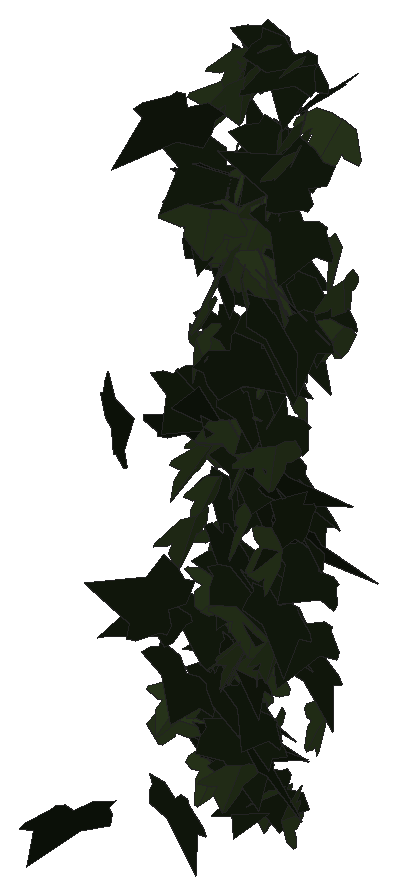
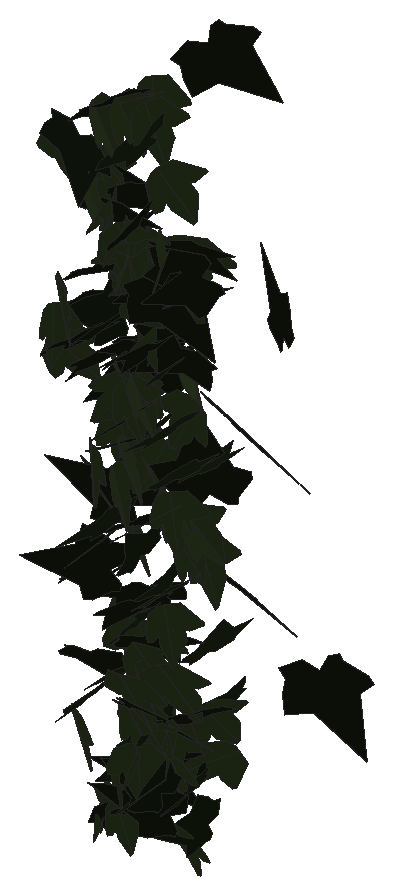
# SketchUp Ruby script. Lengths in inches.
U = 1.inch
M = Sketchup.active_model
def pt(a) = Geom::Point3d.new(a.map { |v| v * U })
def face(e, loops, mat)
  f = e.add_face(loops[0].map { |a| pt(a) })
  loops[1..].each { |l| e.add_face(l.map { |a| pt(a) }).erase! }
  f.material = f.back_material = mat if mat
  f
end
# faces: each face lists its corners as indices into pts; further lists are holes
def faces(e, pts, list, mat = nil) = list.each { |f| face(e, (f[0].is_a?(Array) ? f : [f]).map { |l| l.map { |i| pts[i] } }, mat) }
# xy, xz, yz: faces in a plane at the given z, y or x. An outline is a flat list of corners, or four numbers for a rectangle; further outlines are holes
def ring(l) = l.size == 4 ? [[l[0], l[1]], [l[2], l[1]], [l[2], l[3]], [l[0], l[3]]] : l.each_slice(2).to_a
def flat(e, list, mat, &to3) = list.each { |f| face(e, (f[0].is_a?(Array) ? f : [f]).map { |l| ring(l).map { |u, v| to3.(u, v) } }, mat) }
def xy(e, z, list, mat = nil) = flat(e, list, mat) { |x, y| [x, y, z] }
def xz(e, y, list, mat = nil) = flat(e, list, mat) { |x, z| [x, y, z] }
def yz(e, x, list, mat = nil) = flat(e, list, mat) { |y, z| [x, y, z] }
def lines(e, pts, list) = list.each { |a, b| e.add_line(pt(pts[a]), pt(pts[b])) }
# prism: a flat outline (further loops are holes) pulled along v
def prism(e, loops, v, mat = nil)
  f = face(e, loops, mat); d = Geom::Vector3d.new(v.map { |x| x * U })
  f.pushpull(f.normal.samedirection?(d) ? d.length : -d.length)
end
def box(e, o, s, mat = nil) = prism(e, [[o, [o[0] + s[0], o[1], o[2]], [o[0] + s[0], o[1] + s[1], o[2]], [o[0], o[1] + s[1], o[2]]]], [0, 0, s[2]], mat)
def at(x, y, z, deg = 0) = Geom::Transformation.translation(pt([x, y, z])) * Geom::Transformation.rotation(ORIGIN, Z_AXIS, deg.degrees)
def axes(o, x, y, z) = Geom::Transformation.new([*x, 0, *y, 0, *z, 0, *pt(o).to_a, 1])
def part(name) = M.definitions.add(name)
# library, detail: a bought-in or finely detailed component or shape, given as its bounding box
def library(name, o, s) = part(name).tap { |d| box(d.entities, o, s) }
def detail(e, o, s) = box(e.add_group.entities, o, s)
def put(e, d, t, mat = nil) = e.add_instance(d, t).tap { |i| i.material = mat if mat }
def group(e, t, mat = nil) = e.add_group.tap { |g| g.transformation = t; g.material = mat if mat }.entities
root = M.entities
M.materials.add("1026 AP 7946 SUNNY SIDE UP").color = [254, 231, 186]
M.materials.add("efeu1").color = [18, 25, 13]
M.materials.add("efeu2").color = [43, 57, 29]
c1 = part("ivyleaf_9")
p = [[1.54,2.16,1.25],[1.36,2.04,1.19],[-0.21,0.99,0.68],[-0.71,1.11,0.82],[-0.85,0.86,0.67],[-0.8,0.17,0.21],
  [-0.9,-0.01,0.1],[-0.67,-0.16,-0.02],[-0.08,-0.08,-0.05],[-0.03,-0.6,-0.4],[0.65,-0.88,-0.66],[0.83,-0.6,-0.49],
  [1.29,-0.42,-0.43],[1.8125,-0.07,-0.26],[1.21,0.44,0.15]]
faces(c1.entities,p,[[0,1,2,3,4,5,6,7,8,9,10,11,12,13,14]],"efeu1")
c2 = part("ivyleaf_10")
p = [[0,0.5,-0.03],[-0.0625,2.02,-0.43],[-0.19,2.01,-0.46],[-0.54,1.05,-0.29],[-0.52,0.625,-0.18],[-0.83,0.76,-0.28],
  [-1.16,0.64,-0.33],[-1.15,0.33,-0.24],[-0.77,-0.39,0.02],[-0.3,-0.51,0.16],[0.04,-0.48,0.23],[-0.02,2.01,-0.4375],
  [-0.06,2.01,-0.43],[0.04,-0.49,0.23],[0.67,-0.49,0.14],[1.38,0.36,-0.2],[1.375,0.51,-0.24],[0.81,0.65,-0.19],
  [0.62,0.59,-0.15],[0.6,1.09,-0.28],[0.5,1.23,-0.31]]
faces(c2.entities,p,[[0,1,2,3,4,5,6,7,8,9,10],[11,12,0,13,14,15,16,17,18,19,20]],"efeu2")
put(root,c1,axes([112.36,212.67,281.68],[-0.13343,-0.31321,-0.01587],[0.0925,-0.00204,-0.32907],[0.4842,-0.08592,0.05849]),"1026 AP 7946 SUNNY SIDE UP")
put(root,c1,axes([112.74,212.8,288.39],[0.08903,0.21961,-0.26711],[-0.18165,-0.23608,-0.23226],[-0.50404,0.12387,0.03652]),"1026 AP 7946 SUNNY SIDE UP")
put(root,c2,axes([112.77,212.73,282.15],[-0.39871,-0.07954,0.18483],[-0.22985,-0.12011,-0.26772],[0.20687,-0.28675,0.05877]),"1026 AP 7946 SUNNY SIDE UP")
put(root,c1,axes([112.28,212.46,279.84],[0.33832,-0.23015,0.04396],[0.03121,-0.04159,-0.32451],[0.36711,0.21563,-0.01292]),"1026 AP 7946 SUNNY SIDE UP")
put(root,c2,axes([112.625,212.23,284.41],[0.02229,-0.31208,0.16445],[-0.00199,-0.16158,-0.32269],[0.55246,0.01201,-0.0078]),"1026 AP 7946 SUNNY SIDE UP")
put(root,c1,axes([112.59,212.19,285.28],[-0.22713,-0.19626,0.23409],[-0.02446,-0.24806,-0.23123],[0.47281,-0.10711,0.10049]),"1026 AP 7946 SUNNY SIDE UP")
put(root,c1,axes([112.8,212.52,288.93],[-0.49151,-0.14511,0.04267],[-0.03788,-0.04796,-0.35367],[0.2346,-0.31176,0.03228]),"1026 AP 7946 SUNNY SIDE UP")
put(root,c1,axes([112.56,212.62,288.16],[-0.17816,-0.31965,0.08154],[0.00298,-0.08624,-0.34854],[0.51848,-0.10934,0.03002]),"1026 AP 7946 SUNNY SIDE UP")
put(root,c1,axes([112.32,212.57,288.63],[0.5129,0.04063,0.11681],[0.17107,0.03949,-0.33748],[-0.08046,0.34299,0.02707]),"1026 AP 7946 SUNNY SIDE UP")
put(root,c1,axes([112.39,212.91,287.62],[-0.19443,-0.09617,-0.31279],[0.42257,0.14219,-0.15861],[0.26723,-0.29483,0.02323]),"1026 AP 7946 SUNNY SIDE UP")
put(root,c2,axes([112.74,212.74,283.11],[-0.1662,-0.30756,-0.00442],[0.01182,0.00011,-0.33495],[0.48347,-0.10573,0.00667]),"1026 AP 7946 SUNNY SIDE UP")
put(root,c1,axes([112.48,212.63,280.35],[0.11231,-0.30109,0.06167],[0.01182,-0.06148,-0.31907],[0.48308,0.0715,-0.00653]),"1026 AP 7946 SUNNY SIDE UP")
put(root,c1,axes([112.51,212.91,287.31],[0.02358,-0.30949,0.14387],[0.00979,-0.14128,-0.32004],[0.53495,0.01623,-0.00048]),"1026 AP 7946 SUNNY SIDE UP")
put(root,c1,axes([112.59,212,284.89],[0.47331,0.11972,0.15524],[-0.23704,-0.02521,0.33221],[0.18678,-0.33537,0.02822]),"1026 AP 7946 SUNNY SIDE UP")
put(root,c2,axes([112.84,212.63,290.03],[-0.14622,-0.30283,0.16471],[-0.04767,-0.15953,-0.32688],[0.53763,-0.09651,0.01581]),"1026 AP 7946 SUNNY SIDE UP")
put(root,c2,axes([112.52,211.7,280.51],[-0.14499,-0.12302,-0.29264],[0.36185,0.16992,-0.15215],[0.32404,-0.24479,0.03897]),"1026 AP 7946 SUNNY SIDE UP")
put(root,c2,axes([112.87,212.82,288.15],[-0.50464,-0.10978,0.06791],[-0.07296,-0.06786,-0.34627],[0.18821,-0.32066,0.04785]),"1026 AP 7946 SUNNY SIDE UP")
put(root,c2,axes([112.76,212.4,279.51],[0.42028,-0.18104,0.00491],[-0.01497,-0.02436,-0.33168],[0.28442,0.26624,-0.02472]),"1026 AP 7946 SUNNY SIDE UP")
put(root,c2,axes([112.72,212.27,286.22],[-0.44572,0.16772,-0.0709],[0.07739,-0.05357,-0.33896],[-0.27495,-0.28697,0.01953]),"1026 AP 7946 SUNNY SIDE UP")
put(root,c2,axes([112.84,212.49,284.77],[-0.17448,-0.31481,-0.02675],[0.01254,0.02282,-0.34374],[0.49631,-0.11125,-0.00072]),"1026 AP 7946 SUNNY SIDE UP")
put(root,c1,axes([112.53,212.83,286.27],[0.22125,-0.29308,-0.08379],[0.02449,0.09466,-0.32982],[0.47694,0.1311,0.05581]),"1026 AP 7946 SUNNY SIDE UP")
put(root,c1,axes([112.68,212.62,285.32],[-0.15085,-0.26183,0.18911],[0.03789,-0.1985,-0.27763],[0.50272,-0.06361,0.07767]),"1026 AP 7946 SUNNY SIDE UP")
put(root,c2,axes([112.87,211.6,281.01],[-0.16942,-0.22258,0.21145],[0.01315,-0.22123,-0.24243],[0.47725,-0.07292,0.08175]),"1026 AP 7946 SUNNY SIDE UP")
put(root,c2,axes([112.82,212.24,283.99],[0.01482,-0.29803,0.14397],[0.05323,-0.13988,-0.30678],[0.51599,0.02299,0.02751]),"1026 AP 7946 SUNNY SIDE UP")
put(root,c2,axes([112.78,212.74,287.64],[0.12285,0.33519,-0.00481],[-0.04975,0.00065,-0.35313],[-0.52481,0.0784,0.03235]),"1026 AP 7946 SUNNY SIDE UP")
put(root,c2,axes([112.8125,212.39,281.07],[-0.03901,-0.28735,-0.15112],[0.0832,0.13987,-0.29394],[0.49926,-0.04576,0.03718]),"1026 AP 7946 SUNNY SIDE UP")
put(root,c2,axes([112.9,211.7,283.66],[-0.06475,-0.38216,0.00443],[0.00721,-0.007,-0.39598],[0.60096,-0.04109,0.00523]),"1026 AP 7946 SUNNY SIDE UP")
put(root,c1,axes([112.74,212.9,283.53],[-0.10918,-0.28482,0.14106],[0.01352,-0.14348,-0.30027],[0.49785,-0.05857,0.03909]),"1026 AP 7946 SUNNY SIDE UP")
put(root,c2,axes([112.78,212.87,288.83],[-0.01932,0.08766,-0.34444],[0.04851,-0.33344,-0.09304],[-0.54208,-0.03296,0.00395]),"1026 AP 7946 SUNNY SIDE UP")
put(root,c1,axes([113.07,208.88,280.4],[-0.0023,0.33109,-0.24619],[0.00828,-0.24082,-0.34249],[-0.64374,-0.00428,-0.00353]),"1026 AP 7946 SUNNY SIDE UP")
put(root,c2,axes([112.92,212.51,280.7],[0.44827,-0.14908,0.0037],[-0.01323,-0.02564,-0.33044],[0.23415,0.28396,-0.02576]),"1026 AP 7946 SUNNY SIDE UP")
put(root,c1,axes([113.25,210.88,282.83],[-0.51994,0.12954,0.00606],[-0.0273,-0.03027,-0.3643],[-0.20201,-0.32932,0.03363]),"1026 AP 7946 SUNNY SIDE UP")
put(root,c1,axes([112.75,212.99,287.59],[0.04721,-0.31808,-0.11947],[0.02888,0.11597,-0.32724],[0.53059,0.02199,0.02844]),"1026 AP 7946 SUNNY SIDE UP")
put(root,c1,axes([113.31,212.83,281.53],[-0.46194,0.07247,0.09364],[-0.15939,-0.04098,-0.30548],[-0.08845,-0.30465,0.06145]),"1026 AP 7946 SUNNY SIDE UP")
put(root,c2,axes([113.09,211.87,288.5],[-0.44664,-0.19902,0.03307],[-0.0182,-0.04122,-0.35646],[0.31676,-0.283,0.02615]),"1026 AP 7946 SUNNY SIDE UP")
put(root,c2,axes([112.83,212.04,286.34],[-0.08709,-0.11489,-0.34524],[0.15181,-0.3306,0.09859],[-0.53497,-0.07511,0.08418]),"1026 AP 7946 SUNNY SIDE UP")
put(root,c2,axes([113.1875,212.74,281.46],[0.46257,-0.06588,-0.12299],[-0.17817,0.03822,-0.31011],[0.11836,0.31503,0.01386]),"1026 AP 7946 SUNNY SIDE UP")
put(root,c1,axes([112.97,212.94,287.47],[-0.21006,-0.28712,-0.12868],[0.12665,0.09789,-0.32425],[0.47472,-0.15317,0.02957]),"1026 AP 7946 SUNNY SIDE UP")
put(root,c1,axes([113.16,212.69,282.625],[-0.35266,-0.23229,0.00647],[0.01705,-0.02101,-0.33197],[0.36505,-0.22342,0.02175]),"1026 AP 7946 SUNNY SIDE UP")
put(root,c1,axes([112.74,212.75,279.98],[0.26936,-0.0773,0.26366],[0.34164,-0.13775,-0.19316],[0.24608,0.27585,-0.02043]),"1026 AP 7946 SUNNY SIDE UP")
put(root,c1,axes([112.79,212.88,280.375],[0.19172,-0.17623,0.23619],[0.2556,-0.16532,-0.21998],[0.37757,0.2014,0.02899]),"1026 AP 7946 SUNNY SIDE UP")
put(root,c2,axes([113.22,212.82,280.78],[-0.31728,-0.24219,0.01756],[0.01614,-0.03243,-0.3236],[0.38158,-0.20001,0.02828]),"1026 AP 7946 SUNNY SIDE UP")
put(root,c1,axes([112.95,212.12,281.08],[0.15516,-0.30173,-0.06711],[-0.00335,0.06593,-0.32612],[0.4848,0.09702,0.01923]),"1026 AP 7946 SUNNY SIDE UP")
put(root,c2,axes([113.24,212.48,290.85],[-0.12212,-0.35072,0.04215],[-0.00261,-0.04356,-0.37024],[0.55559,-0.0773,0.00753]),"1026 AP 7946 SUNNY SIDE UP")
put(root,c2,axes([113.28,212.65,282.32],[-0.12128,-0.27246,0.15403],[-0.02122,-0.15256,-0.29145],[0.4894,-0.07414,0.02553]),"1026 AP 7946 SUNNY SIDE UP")
put(root,c1,axes([113.04,212.92,280.25],[0.01083,-0.29283,0.11314],[0.01812,-0.1112,-0.30229],[0.49236,0.01053,0.00864]),"1026 AP 7946 SUNNY SIDE UP")
put(root,c2,axes([113.27,212.93,281.94],[0.46364,-0.07499,-0.09593],[-0.14041,0.02492,-0.31328],[0.12422,0.30808,0.00392]),"1026 AP 7946 SUNNY SIDE UP")
put(root,c2,axes([113.28,212.35,281.53],[0.05512,-0.30794,0.0991],[0.00291,-0.09832,-0.31973],[0.5081,0.03397,-0.00892]),"1026 AP 7946 SUNNY SIDE UP")
put(root,c2,axes([113.23,212.4,287.87],[-0.29873,-0.27787,-0.06803],[0.12113,0.02458,-0.34296],[0.43186,-0.19911,0.04914]),"1026 AP 7946 SUNNY SIDE UP")
put(root,c2,axes([113.3125,212.68,286.57],[0.05917,-0.33716,0.01835],[-0.01161,-0.02066,-0.34948],[0.53094,0.03713,-0.00969]),"1026 AP 7946 SUNNY SIDE UP")
put(root,c2,axes([113.3,212.71,288.43],[-0.07562,-0.32693,-0.09561],[0.03189,0.08893,-0.33983],[0.53264,-0.05174,0.00677]),"1026 AP 7946 SUNNY SIDE UP")
put(root,c2,axes([113.27,212.39,287.87],[-0.04396,-0.31006,-0.15235],[0.07798,0.14141,-0.31806],[0.5333,-0.04623,0.03395]),"1026 AP 7946 SUNNY SIDE UP")
put(root,c2,axes([113.3125,212.59,281.9375],[0.14164,-0.30775,-0.02942],[-0.01765,0.02465,-0.33017],[0.48541,0.09069,-0.00342]),"1026 AP 7946 SUNNY SIDE UP")
put(root,c2,axes([113.33,212.39,281.61],[-0.02341,-0.32444,0.05894],[-0.00696,-0.05891,-0.33493],[0.51849,-0.01544,-0.00183]),"1026 AP 7946 SUNNY SIDE UP")
put(root,c1,axes([113.42,212.86,289],[-0.1915,-0.25398,0.21089],[0.11462,0.19337,0.29093],[-0.50142,0.1412,-0.01403]),"1026 AP 7946 SUNNY SIDE UP")
put(root,c1,axes([113.2,212.83,284.43],[-0.15033,-0.27632,0.15761],[-0.01573,-0.15873,-0.29966],[0.49759,-0.0885,0.03814]),"1026 AP 7946 SUNNY SIDE UP")
put(root,c2,axes([113.45,212.22,287.47],[-0.09713,0.18584,0.30424],[-0.29276,0.23486,-0.19169],[-0.46237,-0.18775,0.05746]),"1026 AP 7946 SUNNY SIDE UP")
put(root,c1,axes([113.09,212.66,281.16],[0.04626,-0.27311,0.1705],[0.05552,-0.16397,-0.28352],[0.50034,0.04345,0.01569]),"1026 AP 7946 SUNNY SIDE UP")
put(root,c2,axes([113.27,212.77,280.71],[-0.0994,0.28042,-0.14587],[-0.01567,-0.14775,-0.29443],[-0.49484,-0.05165,0.03862]),"1026 AP 7946 SUNNY SIDE UP")
put(root,c2,axes([113.37,212.8125,286.51],[-0.08641,-0.33164,0.04672],[0.01379,-0.04927,-0.34618],[0.52655,-0.05314,0.01673]),"1026 AP 7946 SUNNY SIDE UP")
put(root,c1,axes([113.07,212.76,290.69],[0.39409,-0.23362,-0.11272],[-0.05603,0.11792,-0.34699],[0.40086,0.24616,0.06232]),"1026 AP 7946 SUNNY SIDE UP")
put(root,c2,axes([113.4,212.625,281.31],[-0.08924,-0.31739,0.01833],[0.00578,-0.02055,-0.3322],[0.49999,-0.05641,0.00711]),"1026 AP 7946 SUNNY SIDE UP")
put(root,c1,axes([113.28,212.34,280.62],[-0.23194,-0.27794,-0.06798],[0.0569,0.0537,-0.32377],[0.44499,-0.15173,0.00596]),"1026 AP 7946 SUNNY SIDE UP")
put(root,c2,axes([113.46,212.84,289],[-0.23652,-0.30748,0.06986],[-0.00457,-0.07571,-0.35172],[0.49568,-0.14742,0.03009]),"1026 AP 7946 SUNNY SIDE UP")
put(root,c1,axes([113.14,212.16,283.34],[0.25165,-0.2956,-0.03488],[-0.02158,0.02916,-0.34611],[0.46704,0.16062,0.0028]),"1026 AP 7946 SUNNY SIDE UP")
put(root,c1,axes([113.16,209.65,286.19],[-0.00895,0.06325,0.41629],[0.07424,-0.40096,0.06305],[0.63826,0.04752,-0.0015]),"1026 AP 7946 SUNNY SIDE UP")
put(root,c2,axes([113.5,212.35,288.25],[-0.31612,-0.27094,0.06813],[-0.0259,-0.07173,-0.34671],[0.43835,-0.19963,0.02865]),"1026 AP 7946 SUNNY SIDE UP")
put(root,c1,axes([113.29,211.09,281.7],[-0.13524,-0.26955,0.2341],[0.02986,-0.23862,-0.28369],[0.55511,-0.05283,0.07229]),"1026 AP 7946 SUNNY SIDE UP")
put(root,c1,axes([113.01,212.04,280.07],[0.23439,0.02398,0.30058],[0.45901,-0.03482,-0.15097],[0.03181,0.32566,-0.03634]),"1026 AP 7946 SUNNY SIDE UP")
put(root,c2,axes([113.35,212.73,288.78],[0.25869,0.30124,-0.02447],[-0.01508,-0.02377,-0.35372],[-0.47512,0.16477,-0.00209]),"1026 AP 7946 SUNNY SIDE UP")
put(root,c1,axes([113.42,212.59,284.37],[-0.2288,-0.28347,0.10727],[-0.00596,-0.11561,-0.32535],[0.47568,-0.13779,0.04752]),"1026 AP 7946 SUNNY SIDE UP")
put(root,c1,axes([113.24,212.71,283.9375],[0.07631,-0.26117,0.19963],[0.04706,-0.19301,-0.27475],[0.51058,0.05682,-0.00451]),"1026 AP 7946 SUNNY SIDE UP")
put(root,c2,axes([113.42,212.03,285.22],[-0.41145,-0.17797,-0.12311],[0.17403,0.04747,-0.32498],[0.28764,-0.28329,0.02052]),"1026 AP 7946 SUNNY SIDE UP")
put(root,c1,axes([113.6875,210.57,290.98],[-0.0481,0.14973,-0.39135],[0.04897,-0.37983,-0.15869],[-0.64142,-0.04023,0.01723]),"1026 AP 7946 SUNNY SIDE UP")
put(root,c2,axes([113.48,212.83,289.04],[-0.02351,0.28866,-0.20039],[-0.0279,-0.19671,-0.29798],[-0.54806,-0.00237,0.02377]),"1026 AP 7946 SUNNY SIDE UP")
put(root,c2,axes([113.57,212.66,290.91],[-0.01241,-0.34089,0.10394],[0.00773,-0.10295,-0.35181],[0.55982,-0.00613,0.00716]),"1026 AP 7946 SUNNY SIDE UP")
put(root,c2,axes([113.42,212.875,288.73],[-0.18867,0.2635,-0.1972],[0.08189,-0.18745,-0.29824],[-0.50693,-0.12835,0.02521]),"1026 AP 7946 SUNNY SIDE UP")
put(root,c1,axes([113.42,212.95,286.09],[-0.05737,-0.31698,0.10145],[-0.00362,-0.10064,-0.32917],[0.52276,-0.03549,0.00886]),"1026 AP 7946 SUNNY SIDE UP")
put(root,c1,axes([113.34,212.71,287.22],[0.09564,-0.33371,-0.05018],[0.0166,0.04943,-0.34861],[0.5296,0.05871,0.01999]),"1026 AP 7946 SUNNY SIDE UP")
put(root,c2,axes([113.71,212.14,282.28],[-0.50265,-0.1127,0.05506],[-0.06426,-0.04613,-0.34813],[0.18575,-0.32092,0.02856]),"1026 AP 7946 SUNNY SIDE UP")
put(root,c2,axes([113.64,212.72,285.01],[0.08811,-0.33207,-0.0429],[0.00366,0.04069,-0.34657],[0.52586,0.05535,0.0096]),"1026 AP 7946 SUNNY SIDE UP")
put(root,c2,axes([113.67,212.52,285.32],[0.18702,-0.31371,-0.03473],[-0.03947,0.0246,-0.34515],[0.49425,0.12067,-0.01443]),"1026 AP 7946 SUNNY SIDE UP")
put(root,c1,axes([113.49,212.64,282.63],[-0.05762,-0.26341,0.18837],[-0.01488,-0.18458,-0.27472],[0.50532,-0.03547,0.01339]),"1026 AP 7946 SUNNY SIDE UP")
put(root,c2,axes([113.67,211.85,290.8125],[-0.1021,-0.3728,-0.08252],[0.03094,0.07572,-0.38934],[0.59808,-0.06756,0.00606]),"1026 AP 7946 SUNNY SIDE UP")
put(root,c2,axes([113.59,211.05,287.43],[0.23257,-0.33012,0.17709],[-0.08903,0.1649,0.37334],[-0.5798,-0.15774,0.01371]),"1026 AP 7946 SUNNY SIDE UP")
put(root,c1,axes([113.39,212.49,282.17],[0.28678,-0.23526,-0.14043],[-0.03942,0.14734,-0.29859],[0.42466,0.17255,0.06712]),"1026 AP 7946 SUNNY SIDE UP")
put(root,c1,axes([113.42,212.23,285.63],[0.08801,-0.33518,0.05011],[0.0079,-0.0504,-0.35036],[0.53294,0.0561,-0.00308]),"1026 AP 7946 SUNNY SIDE UP")
put(root,c2,axes([113.66,212.57,280.375],[-0.00579,-0.30255,-0.08995],[0.03637,0.08511,-0.31044],[0.49306,-0.00983,0.02185]),"1026 AP 7946 SUNNY SIDE UP")
put(root,c1,axes([113.61,212.37,279.64],[-0.24075,-0.29427,0.08896],[-0.01869,-0.0926,-0.34077],[0.48261,-0.15039,0.03118]),"1026 AP 7946 SUNNY SIDE UP")
put(root,c1,axes([113.8125,212.81,289.39],[-0.53604,-0.06974,-0.04711],[0.07905,-0.02041,-0.35727],[0.10419,-0.3433,0.02871]),"1026 AP 7946 SUNNY SIDE UP")
put(root,c1,axes([113.47,212.51,283],[0.0007,-0.30646,-0.12403],[0.06922,0.11764,-0.31215],[0.51207,-0.01548,0.04236]),"1026 AP 7946 SUNNY SIDE UP")
put(root,c1,axes([113.54,212.03,280.42],[-0.15858,-0.28401,-0.13562],[0.08879,0.11781,-0.30952],[0.48307,-0.11489,0.01237]),"1026 AP 7946 SUNNY SIDE UP")
put(root,c2,axes([113.8,211.59,280.09],[-0.16973,-0.29669,0.05259],[-0.00516,-0.05486,-0.32518],[0.4738,-0.10688,0.0153]),"1026 AP 7946 SUNNY SIDE UP")
put(root,c1,axes([113.64,212.28,280.71],[-0.11641,-0.21899,0.22621],[-0.00776,-0.22614,-0.23406],[0.48895,-0.05572,0.05014]),"1026 AP 7946 SUNNY SIDE UP")
put(root,c1,axes([113.82,212.68,289.49],[-0.32806,-0.26303,0.10434],[-0.08357,-0.08892,-0.34613],[0.43611,-0.21491,0.01216]),"1026 AP 7946 SUNNY SIDE UP")
put(root,c1,axes([113.79,212.74,290.95],[-0.34458,-0.22351,0.18192],[-0.02586,-0.21393,-0.29909],[0.4484,-0.1841,0.12255]),"1026 AP 7946 SUNNY SIDE UP")
put(root,c2,axes([113.69,212.84,289.46],[-0.02411,0.32487,-0.13402],[-0.00819,-0.13226,-0.33564],[-0.55128,-0.01224,0.01085]),"1026 AP 7946 SUNNY SIDE UP")
put(root,c2,axes([113.49,212.21,287.72],[-0.35981,0.01767,-0.27521],[0.3837,-0.13112,-0.22495],[-0.17358,-0.32648,0.07323]),"1026 AP 7946 SUNNY SIDE UP")
put(root,c2,axes([113.78,211.91,285.01],[0.22741,-0.29837,0.0892],[0.02594,-0.08986,-0.34125],[0.48858,0.14365,-0.0234]),"1026 AP 7946 SUNNY SIDE UP")
put(root,c2,axes([113.66,212.4,286.33],[-0.34639,-0.18425,-0.18783],[0.27691,0.06735,-0.2906],[0.29749,-0.27722,0.0518]),"1026 AP 7946 SUNNY SIDE UP")
put(root,c1,axes([113.62,211.75,286.6],[0.01286,-0.06768,-0.39876],[0.01352,0.38671,-0.06727],[0.61712,-0.00706,0.00978]),"1026 AP 7946 SUNNY SIDE UP")
put(root,c1,axes([113.64,212.02,282.96],[-0.05902,-0.28407,-0.17306],[0.09666,0.15846,-0.29209],[0.50854,-0.06309,0.03543]),"1026 AP 7946 SUNNY SIDE UP")
put(root,c2,axes([113.89,212.85,289.8],[0.05483,-0.34349,-0.07407],[0.00196,0.07041,-0.35517],[0.55119,0.03392,0.00863]),"1026 AP 7946 SUNNY SIDE UP")
put(root,c1,axes([113.9,212.51,285.38],[-0.3226,-0.20879,0.17497],[-0.06115,-0.18972,-0.28777],[0.41995,-0.18801,0.09251]),"1026 AP 7946 SUNNY SIDE UP")
put(root,c2,axes([113.91,212.33,279.45],[-0.07536,-0.30387,0.02634],[0.00145,-0.02777,-0.31704],[0.47973,-0.04765,0.00509]),"1026 AP 7946 SUNNY SIDE UP")
put(root,c2,axes([113.9,212.79,290.78],[0.07331,-0.35113,0.04697],[-0.00043,-0.04803,-0.36513],[0.55716,0.04617,-0.00646]),"1026 AP 7946 SUNNY SIDE UP")
put(root,c2,axes([113.83,212.375,286.44],[0.37032,-0.23244,0.08063],[0.05877,-0.07507,-0.34024],[0.38183,0.23699,-0.02583]),"1026 AP 7946 SUNNY SIDE UP")
put(root,c1,axes([113.71,212.94,287.5625],[0.02245,-0.33983,0.01349],[-0.00032,-0.01505,-0.35049],[0.53487,0.01425,-0.00077]),"1026 AP 7946 SUNNY SIDE UP")
put(root,c1,axes([114.02,212.35,279.57],[-0.04628,-0.09694,-0.3193],[0.05431,-0.30984,0.09481],[-0.50691,-0.02434,0.03931]),"1026 AP 7946 SUNNY SIDE UP")
put(root,c1,axes([113.63,212.75,284.44],[0.31953,-0.24869,-0.10646],[-0.0209,0.11832,-0.32402],[0.42209,0.19412,0.06455]),"1026 AP 7946 SUNNY SIDE UP")
put(root,c2,axes([113.97,212.91,289.65],[0.12096,-0.33439,0.06587],[0.0004,-0.06744,-0.35356],[0.53589,0.07553,-0.01461]),"1026 AP 7946 SUNNY SIDE UP")
put(root,c2,axes([113.99,211.5,284.15],[0.21424,-0.30301,-0.03701],[-0.01785,0.0324,-0.34207],[0.47916,0.13669,0.00381]),"1026 AP 7946 SUNNY SIDE UP")
put(root,c1,axes([113.71,212.09,280.24],[0.32616,-0.25483,-0.00065],[-0.02071,-0.01177,-0.33808],[0.40017,0.20709,-0.01697]),"1026 AP 7946 SUNNY SIDE UP")
put(root,c1,axes([113.88,212.73,290.94],[-0.15008,-0.33875,0.0568],[-0.00568,-0.05822,-0.36269],[0.54013,-0.09474,0.01197]),"1026 AP 7946 SUNNY SIDE UP")
put(root,c2,axes([113.96,212.84,285.3125],[0.29949,-0.2693,-0.06867],[0.04927,0.09946,-0.3287],[0.43286,0.175,0.08493]),"1026 AP 7946 SUNNY SIDE UP")
put(root,c1,axes([113.76,210.28,280.21],[0.10009,-0.3275,0.12404],[0.03345,-0.12041,-0.3444],[0.54865,0.06709,-0.00163]),"1026 AP 7946 SUNNY SIDE UP")
put(root,c1,axes([113.99,212.78,288.32],[-0.21487,-0.29728,0.10228],[-0.01229,-0.10686,-0.33566],[0.49352,-0.13209,0.03617]),"1026 AP 7946 SUNNY SIDE UP")
put(root,c1,axes([114.52,209.1,284.05],[-0.34317,0.28173,0.22656],[-0.26986,0.1413,-0.36376],[-0.49118,-0.27446,0.04156]),"1026 AP 7946 SUNNY SIDE UP")
put(root,c1,axes([114.22,212.86,290.3125],[0.05332,0.32828,0.13405],[-0.01997,0.1299,-0.33831],[-0.55382,0.02692,0.02511]),"1026 AP 7946 SUNNY SIDE UP")
put(root,c1,axes([114.11,212.6875,282.05],[-0.39475,-0.18488,-0.06342],[0.11314,0.00353,-0.31863],[0.28418,-0.25821,0.03877]),"1026 AP 7946 SUNNY SIDE UP")
put(root,c2,axes([114.36,211.8125,287.58],[-0.14775,0.14481,-0.35088],[-0.26424,0.29734,0.17931],[0.51983,0.1923,-0.00858]),"1026 AP 7946 SUNNY SIDE UP")
put(root,c1,axes([113.94,212.9,283.9],[0.06492,-0.3218,0.03567],[0.00002,-0.03675,-0.33441],[0.50923,0.04103,-0.00454]),"1026 AP 7946 SUNNY SIDE UP")
put(root,c1,axes([113.9,212.59,286.92],[0.09176,-0.31875,-0.13285],[0.03074,0.13185,-0.33051],[0.53874,0.04677,0.04149]),"1026 AP 7946 SUNNY SIDE UP")
put(root,c2,axes([114.24,212.23,289.67],[-0.01751,-0.34842,-0.00421],[0.01073,0.00189,-0.35904],[0.54776,-0.01118,0.0069]),"1026 AP 7946 SUNNY SIDE UP")
put(root,c2,axes([114.35,211.66,283.73],[0.27586,-0.27286,-0.20815],[-0.1898,0.16058,-0.333],[0.49745,0.21259,-0.01163]),"1026 AP 7946 SUNNY SIDE UP")
put(root,c1,axes([114.67,211.99,289.49],[-0.29062,0.19585,0.25871],[-0.36755,0.11194,-0.2677],[-0.33807,-0.29007,0.06864]),"1026 AP 7946 SUNNY SIDE UP")
put(root,c2,axes([114.34,212.08,279.32],[-0.02421,0.10473,0.32836],[-0.23704,0.28223,-0.10158],[-0.4703,-0.14764,0.03429]),"1026 AP 7946 SUNNY SIDE UP")
put(root,c1,axes([113.8,212.26,284.38],[0.18712,-0.08699,0.31702],[0.43874,-0.13324,-0.1505],[0.24719,0.30234,0.02714]),"1026 AP 7946 SUNNY SIDE UP")
put(root,c2,axes([114.3125,211.77,285.26],[-0.22712,-0.31444,-0.02354],[0.01995,0.01735,-0.35635],[0.49513,-0.14493,0.00356]),"1026 AP 7946 SUNNY SIDE UP")
put(root,c1,axes([113.88,212.36,287.39],[0.33845,-0.22001,0.15714],[0.17429,-0.10668,-0.31768],[0.38441,0.24207,0.00568]),"1026 AP 7946 SUNNY SIDE UP")
put(root,c1,axes([114.07,212.89,281.42],[0.08745,-0.31189,0.03143],[0.01019,-0.03164,-0.32656],[0.49294,0.05599,0.00118]),"1026 AP 7946 SUNNY SIDE UP")
put(root,c2,axes([114.35,211.75,282.26],[-0.00265,-0.33707,-0.02247],[0.01224,0.01985,-0.34705],[0.53079,-0.00214,0.00789]),"1026 AP 7946 SUNNY SIDE UP")
put(root,c1,axes([114.23,212.96,287.17],[-0.11477,-0.32537,0.05811],[-0.00691,-0.0587,-0.34376],[0.5197,-0.07264,0.00826]),"1026 AP 7946 SUNNY SIDE UP")
put(root,c1,axes([113.92,212.62,283.43],[0.38443,-0.09995,0.20711],[0.29752,-0.06983,-0.27245],[0.19153,0.3091,0.00751]),"1026 AP 7946 SUNNY SIDE UP")
put(root,c2,axes([114.42,213,287.875],[0.24943,-0.29295,-0.07411],[-0.00032,0.07932,-0.34064],[0.4737,0.15431,0.03879]),"1026 AP 7946 SUNNY SIDE UP")
put(root,c1,axes([114.57,212.04,284.37],[-0.46294,0.12788,-0.20001],[0.2594,-0.10747,-0.33004],[-0.25892,-0.33631,0.02696]),"1026 AP 7946 SUNNY SIDE UP")
put(root,c2,axes([114.51,212.51,280.76],[0.26725,-0.25257,-0.1029],[-0.05958,0.09293,-0.31244],[0.42206,0.17304,0.02105]),"1026 AP 7946 SUNNY SIDE UP")
put(root,c1,axes([114.48,212.49,283.13],[-0.24302,-0.1954,0.22035],[-0.04907,-0.23095,-0.2407],[0.45418,-0.1295,0.0919]),"1026 AP 7946 SUNNY SIDE UP")
put(root,c2,axes([114.61,212.72,286.8125],[-0.17287,-0.24083,0.21951],[-0.06031,-0.21519,-0.27048],[0.50345,-0.10847,0.04297]),"1026 AP 7946 SUNNY SIDE UP")
put(root,c2,axes([114.51,212.83,289.97],[0.52286,-0.11119,-0.03894],[-0.07094,-0.01819,-0.35987],[0.17015,0.3341,-0.03038]),"1026 AP 7946 SUNNY SIDE UP")
put(root,c2,axes([114.54,212.99,287.41],[-0.04804,-0.3264,-0.08985],[0.06526,0.08143,-0.33557],[0.52646,-0.03988,0.03339]),"1026 AP 7946 SUNNY SIDE UP")
put(root,c1,axes([114.33,211.74,287.43],[0.09639,-0.34396,0.05562],[0.00552,-0.05619,-0.3602],[0.54792,0.06108,-0.00615]),"1026 AP 7946 SUNNY SIDE UP")
put(root,c1,axes([114.44,211.73,282.86],[-0.02812,-0.32147,0.07829],[0.0059,-0.07813,-0.33204],[0.52005,-0.0165,0.008]),"1026 AP 7946 SUNNY SIDE UP")
put(root,c1,axes([114.47,211.89,287.36],[-0.14982,-0.36597,-0.04494],[0.03712,0.03676,-0.38912],[0.57795,-0.09723,0.01334]),"1026 AP 7946 SUNNY SIDE UP")
